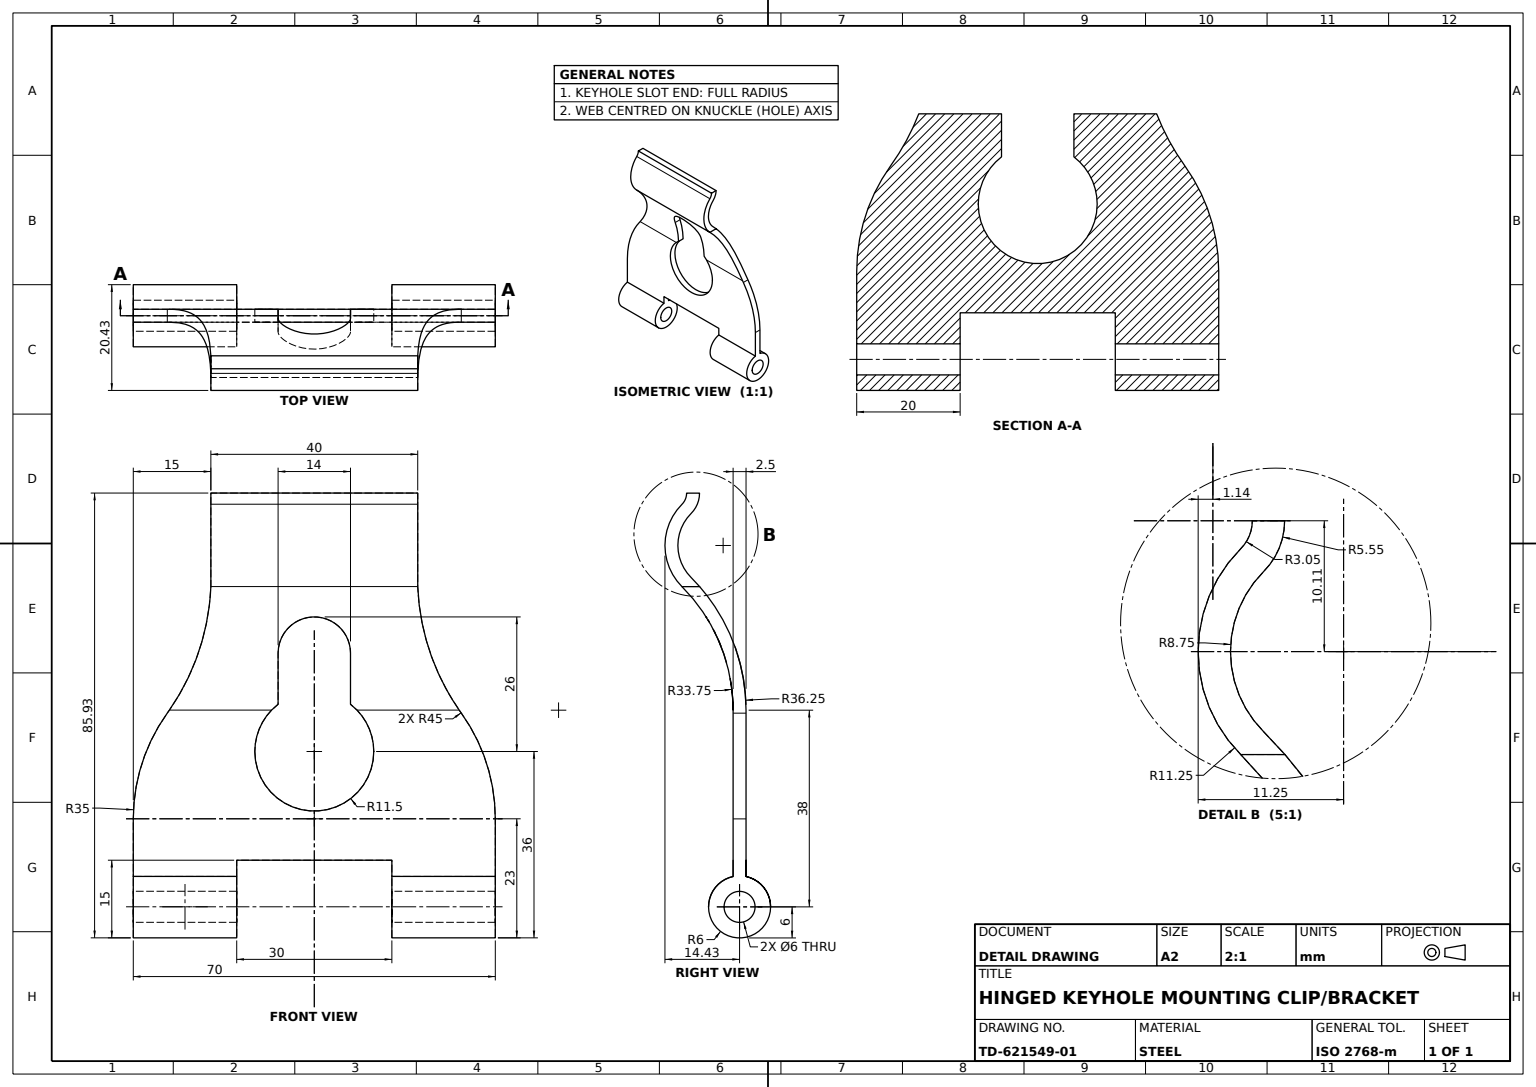
ISO-10303-21;
HEADER;
FILE_DESCRIPTION((''),'2;1');
FILE_NAME('','',(''),(''),'','','');
FILE_SCHEMA(('AUTOMOTIVE_DESIGN'));
ENDSEC;
DATA;
#1=APPLICATION_CONTEXT('');
#2=PRODUCT_CONTEXT('',#1,'mechanical');
#3=PRODUCT('','','',(#2));
#4=PRODUCT_DEFINITION_FORMATION('','',#3);
#5=PRODUCT_DEFINITION_CONTEXT('',#1,'design');
#6=PRODUCT_DEFINITION('','',#4,#5);
#7=PRODUCT_DEFINITION_SHAPE('','',#6);
#8=(LENGTH_UNIT()NAMED_UNIT(*)SI_UNIT(.MILLI.,.METRE.));
#9=(NAMED_UNIT(*)PLANE_ANGLE_UNIT()SI_UNIT($,.RADIAN.));
#10=(NAMED_UNIT(*)SI_UNIT($,.STERADIAN.)SOLID_ANGLE_UNIT());
#11=UNCERTAINTY_MEASURE_WITH_UNIT(LENGTH_MEASURE(1.E-05),#8,'distance_accuracy_value','');
#12=(GEOMETRIC_REPRESENTATION_CONTEXT(3)GLOBAL_UNCERTAINTY_ASSIGNED_CONTEXT((#11))GLOBAL_UNIT_ASSIGNED_CONTEXT((#8,#9,#10))REPRESENTATION_CONTEXT('',''));
#13=CARTESIAN_POINT('',(15.,0.,6.));
#14=VERTEX_POINT('',#13);
#15=CARTESIAN_POINT('',(15.,5.868347,1.25));
#16=VERTEX_POINT('',#15);
#17=CARTESIAN_POINT('',(15.,0.,0.));
#18=DIRECTION('',(-1.,0.,0.));
#19=DIRECTION('',(0.,-1.,0.));
#20=AXIS2_PLACEMENT_3D('',#17,#18,#19);
#21=CIRCLE('',#20,6.);
#22=EDGE_CURVE('',#14,#16,#21,.T.);
#23=ORIENTED_EDGE('',*,*,#22,.F.);
#24=CARTESIAN_POINT('',(35.,0.,6.));
#25=VERTEX_POINT('',#24);
#26=VECTOR('',#18,1000.);
#27=LINE('',#24,#26);
#28=EDGE_CURVE('',#25,#14,#27,.T.);
#29=ORIENTED_EDGE('',*,*,#28,.F.);
#30=CARTESIAN_POINT('',(35.,5.868347,1.25));
#31=VERTEX_POINT('',#30);
#32=CARTESIAN_POINT('',(35.,0.,0.));
#33=DIRECTION('',(1.,0.,0.));
#34=DIRECTION('',(0.,0.,-1.));
#35=AXIS2_PLACEMENT_3D('',#32,#33,#34);
#36=CIRCLE('',#35,6.);
#37=EDGE_CURVE('',#31,#25,#36,.T.);
#38=ORIENTED_EDGE('',*,*,#37,.F.);
#39=LINE('',#30,#26);
#40=EDGE_CURVE('',#31,#16,#39,.T.);
#41=ORIENTED_EDGE('',*,*,#40,.T.);
#42=EDGE_LOOP('',(#23,#29,#38,#41));
#43=FACE_OUTER_BOUND('',#42,.T.);
#44=DIRECTION('',(0.,0.,1.));
#45=AXIS2_PLACEMENT_3D('',#32,#18,#44);
#46=CYLINDRICAL_SURFACE('',#45,6.);
#47=ADVANCED_FACE('',(#43),#46,.T.);
#48=CARTESIAN_POINT('',(-15.,0.,-3.));
#49=VERTEX_POINT('',#48);
#50=CARTESIAN_POINT('',(-15.,0.,3.));
#51=VERTEX_POINT('',#50);
#52=CARTESIAN_POINT('',(-15.,0.,0.));
#53=AXIS2_PLACEMENT_3D('',#52,#33,#34);
#54=CIRCLE('',#53,3.);
#55=EDGE_CURVE('',#49,#51,#54,.T.);
#56=ORIENTED_EDGE('',*,*,#55,.F.);
#57=EDGE_CURVE('',#51,#49,#54,.T.);
#58=ORIENTED_EDGE('',*,*,#57,.F.);
#59=EDGE_LOOP('',(#56,#58));
#60=FACE_BOUND('',#59,.T.);
#61=CARTESIAN_POINT('',(-15.,5.868347,1.25));
#62=VERTEX_POINT('',#61);
#63=CARTESIAN_POINT('',(-15.,0.,6.));
#64=VERTEX_POINT('',#63);
#65=CIRCLE('',#53,6.);
#66=EDGE_CURVE('',#62,#64,#65,.T.);
#67=ORIENTED_EDGE('',*,*,#66,.T.);
#68=CARTESIAN_POINT('',(-15.,0.,-6.));
#69=VERTEX_POINT('',#68);
#70=EDGE_CURVE('',#64,#69,#65,.T.);
#71=ORIENTED_EDGE('',*,*,#70,.T.);
#72=CARTESIAN_POINT('',(-15.,5.868347,-1.25));
#73=VERTEX_POINT('',#72);
#74=EDGE_CURVE('',#69,#73,#65,.T.);
#75=ORIENTED_EDGE('',*,*,#74,.T.);
#76=CARTESIAN_POINT('',(-15.,9.,-1.25));
#77=VERTEX_POINT('',#76);
#78=DIRECTION('',(0.,1.,0.));
#79=VECTOR('',#78,1000.);
#80=LINE('',#72,#79);
#81=EDGE_CURVE('',#73,#77,#80,.T.);
#82=ORIENTED_EDGE('',*,*,#81,.T.);
#83=CARTESIAN_POINT('',(-15.,9.,1.25));
#84=VERTEX_POINT('',#83);
#85=CARTESIAN_POINT('',(-15.,9.,-6.));
#86=VECTOR('',#44,1000.);
#87=LINE('',#85,#86);
#88=EDGE_CURVE('',#77,#84,#87,.T.);
#89=ORIENTED_EDGE('',*,*,#88,.T.);
#90=VECTOR('',#19,1000.);
#91=LINE('',#61,#90);
#92=EDGE_CURVE('',#84,#62,#91,.T.);
#93=ORIENTED_EDGE('',*,*,#92,.T.);
#94=EDGE_LOOP('',(#67,#71,#75,#82,#89,#93));
#95=FACE_OUTER_BOUND('',#94,.T.);
#96=CARTESIAN_POINT('',(-15.,-6.,-6.));
#97=AXIS2_PLACEMENT_3D('',#96,#33,#34);
#98=PLANE('',#97);
#99=ADVANCED_FACE('',(#60,#95),#98,.T.);
#100=ORIENTED_EDGE('',*,*,#70,.F.);
#101=CARTESIAN_POINT('',(-35.,0.,6.));
#102=VERTEX_POINT('',#101);
#103=EDGE_CURVE('',#64,#102,#27,.T.);
#104=ORIENTED_EDGE('',*,*,#103,.T.);
#105=CARTESIAN_POINT('',(-35.,0.,-6.));
#106=VERTEX_POINT('',#105);
#107=CARTESIAN_POINT('',(-35.,0.,0.));
#108=AXIS2_PLACEMENT_3D('',#107,#33,#34);
#109=CIRCLE('',#108,6.);
#110=EDGE_CURVE('',#102,#106,#109,.T.);
#111=ORIENTED_EDGE('',*,*,#110,.T.);
#112=CARTESIAN_POINT('',(35.,0.,-6.));
#113=LINE('',#112,#26);
#114=EDGE_CURVE('',#69,#106,#113,.T.);
#115=ORIENTED_EDGE('',*,*,#114,.F.);
#116=EDGE_LOOP('',(#100,#104,#111,#115));
#117=FACE_OUTER_BOUND('',#116,.T.);
#118=ADVANCED_FACE('',(#117),#46,.T.);
#119=CARTESIAN_POINT('',(7.,49.,3.092908));
#120=VERTEX_POINT('',#119);
#121=CARTESIAN_POINT('',(7.,39.124144,1.268727));
#122=VERTEX_POINT('',#121);
#123=CARTESIAN_POINT('',(7.,38.,35.));
#124=AXIS2_PLACEMENT_3D('',#123,#18,#78);
#125=CIRCLE('',#124,33.75);
#126=EDGE_CURVE('',#120,#122,#125,.T.);
#127=ORIENTED_EDGE('',*,*,#126,.T.);
#128=CARTESIAN_POINT('',(8.261356,38.,1.25));
#129=VERTEX_POINT('',#128);
#130=CARTESIAN_POINT('',(7.448007,38.780435,1.257272));
#131=CARTESIAN_POINT('',(7.868457,38.405735,1.25));
#132=B_SPLINE_CURVE_WITH_KNOTS('',3,(#121,#130,#131,#128),.UNSPECIFIED.,.F.,.F.,(4,4),(0.,0.001689695),.UNSPECIFIED.);
#133=EDGE_CURVE('',#122,#129,#132,.T.);
#134=ORIENTED_EDGE('',*,*,#133,.T.);
#135=CARTESIAN_POINT('',(28.015673,38.,1.25));
#136=VERTEX_POINT('',#135);
#137=CARTESIAN_POINT('',(35.,38.,1.25));
#138=LINE('',#137,#26);
#139=EDGE_CURVE('',#136,#129,#138,.T.);
#140=ORIENTED_EDGE('',*,*,#139,.F.);
#141=CARTESIAN_POINT('',(20.,61.864854,11.135146));
#142=VERTEX_POINT('',#141);
#143=CARTESIAN_POINT('',(20.067704,60.195455,9.465747));
#144=CARTESIAN_POINT('',(20.233479,58.385184,8.002505));
#145=CARTESIAN_POINT('',(20.628542,55.962208,6.421049));
#146=CARTESIAN_POINT('',(20.717007,55.469533,6.117247));
#147=CARTESIAN_POINT('',(20.914793,54.468142,5.534795));
#148=CARTESIAN_POINT('',(21.024568,53.957601,5.255257));
#149=CARTESIAN_POINT('',(21.38398,52.420105,4.463923));
#150=CARTESIAN_POINT('',(21.663718,51.385624,3.997756));
#151=CARTESIAN_POINT('',(22.310298,49.303225,3.179391));
#152=CARTESIAN_POINT('',(22.677119,48.255291,2.827222));
#153=CARTESIAN_POINT('',(23.298532,46.676942,2.37988));
#154=CARTESIAN_POINT('',(23.517542,46.149748,2.24427));
#155=CARTESIAN_POINT('',(23.980432,45.09379,1.999479));
#156=CARTESIAN_POINT('',(24.224013,44.565913,1.890595));
#157=CARTESIAN_POINT('',(25.490165,41.956451,1.415609));
#158=CARTESIAN_POINT('',(26.66763,39.93888,1.25));
#159=B_SPLINE_CURVE_WITH_KNOTS('',3,(#141,#143,#144,#145,#146,#147,#148,#149,#150,#151,#152,#153,#154,#155,#156,#157,#158,#135),.UNSPECIFIED.,.F.,.F.,(4,2,2,2,2,2,2,2,4),(0.,0.006991698,0.008739623,0.010487547,0.013983397,0.017479246,0.01922717,0.020975095,0.027966793),.UNSPECIFIED.);
#160=EDGE_CURVE('',#142,#136,#159,.T.);
#161=ORIENTED_EDGE('',*,*,#160,.F.);
#162=CARTESIAN_POINT('',(-20.,61.864854,11.135146));
#163=VERTEX_POINT('',#162);
#164=CARTESIAN_POINT('',(35.,61.864854,11.135146));
#165=LINE('',#164,#26);
#166=EDGE_CURVE('',#142,#163,#165,.T.);
#167=ORIENTED_EDGE('',*,*,#166,.T.);
#168=CARTESIAN_POINT('',(-28.015673,38.,1.25));
#169=VERTEX_POINT('',#168);
#170=CARTESIAN_POINT('',(-26.66803,39.938305,1.25));
#171=CARTESIAN_POINT('',(-25.494861,41.949522,1.415707));
#172=CARTESIAN_POINT('',(-24.235569,44.541424,1.885806));
#173=CARTESIAN_POINT('',(-23.994118,45.063713,1.993062));
#174=CARTESIAN_POINT('',(-23.531942,46.115821,2.235882));
#175=CARTESIAN_POINT('',(-23.310498,46.647516,2.371999));
#176=CARTESIAN_POINT('',(-22.683251,48.237849,2.821393));
#177=CARTESIAN_POINT('',(-22.314887,49.289626,3.174576));
#178=CARTESIAN_POINT('',(-21.667657,51.371771,3.991791));
#179=CARTESIAN_POINT('',(-21.388816,52.402154,4.455803));
#180=CARTESIAN_POINT('',(-21.031209,53.927873,5.239418));
#181=CARTESIAN_POINT('',(-20.922125,54.43313,5.515242));
#182=CARTESIAN_POINT('',(-20.723185,55.436284,6.09715));
#183=CARTESIAN_POINT('',(-20.633244,55.935017,6.403886));
#184=CARTESIAN_POINT('',(-20.233612,58.377977,7.99553));
#185=CARTESIAN_POINT('',(-20.067728,60.194856,9.465148));
#186=B_SPLINE_CURVE_WITH_KNOTS('',3,(#168,#170,#171,#172,#173,#174,#175,#176,#177,#178,#179,#180,#181,#182,#183,#184,#185,#162),.UNSPECIFIED.,.F.,.F.,(4,2,2,2,2,2,2,2,4),(0.,0.006992736,0.00874092,0.010489104,0.013985472,0.01748184,0.019230024,0.020978208,0.027970943),.UNSPECIFIED.);
#187=EDGE_CURVE('',#169,#163,#186,.T.);
#188=ORIENTED_EDGE('',*,*,#187,.F.);
#189=CARTESIAN_POINT('',(-8.261356,38.,1.25));
#190=VERTEX_POINT('',#189);
#191=EDGE_CURVE('',#190,#169,#138,.T.);
#192=ORIENTED_EDGE('',*,*,#191,.F.);
#193=CARTESIAN_POINT('',(-7.,39.124144,1.268727));
#194=VERTEX_POINT('',#193);
#195=CARTESIAN_POINT('',(-7.868457,38.405735,1.25));
#196=CARTESIAN_POINT('',(-7.448007,38.780435,1.257272));
#197=B_SPLINE_CURVE_WITH_KNOTS('',3,(#189,#195,#196,#193),.UNSPECIFIED.,.F.,.F.,(4,4),(0.,0.001689695),.UNSPECIFIED.);
#198=EDGE_CURVE('',#190,#194,#197,.T.);
#199=ORIENTED_EDGE('',*,*,#198,.T.);
#200=CARTESIAN_POINT('',(-7.,49.,3.092908));
#201=VERTEX_POINT('',#200);
#202=CARTESIAN_POINT('',(-7.,38.,35.));
#203=AXIS2_PLACEMENT_3D('',#202,#33,#19);
#204=CIRCLE('',#203,33.75);
#205=EDGE_CURVE('',#194,#201,#204,.T.);
#206=ORIENTED_EDGE('',*,*,#205,.T.);
#207=CARTESIAN_POINT('',(-7.,49.459493,3.251319));
#208=CARTESIAN_POINT('',(-6.955225,49.908016,3.417036));
#209=CARTESIAN_POINT('',(-6.826304,50.565722,3.675559));
#210=CARTESIAN_POINT('',(-6.772953,50.78243,3.763389));
#211=CARTESIAN_POINT('',(-6.645453,51.210861,3.942158));
#212=CARTESIAN_POINT('',(-6.570874,51.423584,4.033545));
#213=CARTESIAN_POINT('',(-6.31836,52.046131,4.308397));
#214=CARTESIAN_POINT('',(-6.11307,52.439076,4.491852));
#215=CARTESIAN_POINT('',(-5.750706,52.997324,4.764496));
#216=CARTESIAN_POINT('',(-5.620776,53.178174,4.854944));
#217=CARTESIAN_POINT('',(-5.341893,53.529287,5.03431));
#218=CARTESIAN_POINT('',(-5.192379,53.699984,5.123477));
#219=CARTESIAN_POINT('',(-4.723451,54.185711,5.382103));
#220=CARTESIAN_POINT('',(-4.381504,54.478099,5.544528));
#221=CARTESIAN_POINT('',(-3.821821,54.869026,5.767809));
#222=CARTESIAN_POINT('',(-3.627407,54.991332,5.838817));
#223=CARTESIAN_POINT('',(-3.221534,55.218992,5.972664));
#224=CARTESIAN_POINT('',(-3.010536,55.323866,6.035227));
#225=CARTESIAN_POINT('',(-2.367891,55.6039,6.203946));
#226=CARTESIAN_POINT('',(-1.921495,55.747942,6.29309));
#227=CARTESIAN_POINT('',(-1.222655,55.896509,6.385653));
#228=CARTESIAN_POINT('',(-0.983157,55.934845,6.409708));
#229=CARTESIAN_POINT('',(-0.501467,55.986215,6.441998));
#230=CARTESIAN_POINT('',(-0.26109,55.999242,6.450223));
#231=CARTESIAN_POINT('',(0.21875,56.000694,6.451138));
#232=CARTESIAN_POINT('',(0.458214,55.989116,6.443827));
#233=CARTESIAN_POINT('',(0.936227,55.941266,6.41374));
#234=CARTESIAN_POINT('',(1.176202,55.904679,6.390766));
#235=CARTESIAN_POINT('',(1.884086,55.758874,6.29986));
#236=CARTESIAN_POINT('',(2.335046,55.615791,6.211226));
#237=CARTESIAN_POINT('',(2.982968,55.33697,6.043071));
#238=CARTESIAN_POINT('',(3.195077,55.232627,5.980761));
#239=CARTESIAN_POINT('',(3.601997,55.006645,5.847749));
#240=CARTESIAN_POINT('',(3.797576,54.884796,5.776915));
#241=CARTESIAN_POINT('',(4.173959,54.624098,5.627829));
#242=CARTESIAN_POINT('',(4.35476,54.485245,5.549575));
#243=CARTESIAN_POINT('',(4.702032,54.19064,5.386591));
#244=CARTESIAN_POINT('',(4.869045,54.034225,5.301517));
#245=CARTESIAN_POINT('',(5.340682,53.547659,5.042231));
#246=CARTESIAN_POINT('',(5.618752,53.19864,4.863034));
#247=CARTESIAN_POINT('',(6.106229,52.451511,4.497717));
#248=CARTESIAN_POINT('',(6.315978,52.050643,4.310508));
#249=CARTESIAN_POINT('',(6.651425,51.226332,3.946342));
#250=CARTESIAN_POINT('',(6.779579,50.799961,3.767828));
#251=CARTESIAN_POINT('',(6.954259,49.916967,3.420362));
#252=CARTESIAN_POINT('',(7.,49.46001,3.251497));
#253=B_SPLINE_CURVE_WITH_KNOTS('',3,(#200,#207,#208,#209,#210,#211,#212,#213,#214,#215,#216,#217,#218,#219,#220,#221,#222,#223,#224,#225,#226,#227,#228,#229,#230,#231,#232,#233,#234,#235,#236,#237,#238,#239,#240,#241,#242,#243,#244,#245,#246,#247,#248,#249,#250,#251,#252,#119),.UNSPECIFIED.,.F.,.F.,(4,2,2,2,2,2,2,2,2,2,2,2,2,2,2,2,2,2,2,2,2,2,2,4),(0.,0.00143658,0.00215487,0.00287316,0.004309739,0.005028029,0.005746319,0.007182899,0.007901189,0.008619479,0.010056058,0.010774348,0.011492638,0.012210928,0.012929218,0.014365798,0.015084088,0.015802378,0.016520667,0.017238957,0.018675537,0.020112117,0.021548697,0.022985276),.UNSPECIFIED.);
#254=EDGE_CURVE('',#201,#120,#253,.T.);
#255=ORIENTED_EDGE('',*,*,#254,.T.);
#256=EDGE_LOOP('',(#127,#134,#140,#161,#167,#188,#192,#199,#206,#255));
#257=FACE_OUTER_BOUND('',#256,.T.);
#258=CARTESIAN_POINT('',(35.,38.,35.));
#259=AXIS2_PLACEMENT_3D('',#258,#18,#44);
#260=CYLINDRICAL_SURFACE('',#259,33.75);
#261=ADVANCED_FACE('',(#257),#260,.F.);
#262=CARTESIAN_POINT('',(-20.,77.774756,11.135146));
#263=VERTEX_POINT('',#262);
#264=CARTESIAN_POINT('',(-20.,79.931432,10.241822));
#265=VERTEX_POINT('',#264);
#266=CARTESIAN_POINT('',(-20.,79.931432,13.291822));
#267=AXIS2_PLACEMENT_3D('',#266,#33,#19);
#268=CIRCLE('',#267,3.05);
#269=EDGE_CURVE('',#263,#265,#268,.T.);
#270=ORIENTED_EDGE('',*,*,#269,.F.);
#271=CARTESIAN_POINT('',(20.,77.774756,11.135146));
#272=VERTEX_POINT('',#271);
#273=CARTESIAN_POINT('',(35.,77.774756,11.135146));
#274=LINE('',#273,#26);
#275=EDGE_CURVE('',#272,#263,#274,.T.);
#276=ORIENTED_EDGE('',*,*,#275,.F.);
#277=CARTESIAN_POINT('',(20.,79.931432,10.241822));
#278=VERTEX_POINT('',#277);
#279=CARTESIAN_POINT('',(20.,79.931432,13.291822));
#280=AXIS2_PLACEMENT_3D('',#279,#18,#34);
#281=CIRCLE('',#280,3.05);
#282=EDGE_CURVE('',#278,#272,#281,.T.);
#283=ORIENTED_EDGE('',*,*,#282,.F.);
#284=CARTESIAN_POINT('',(35.,79.931432,10.241822));
#285=LINE('',#284,#26);
#286=EDGE_CURVE('',#278,#265,#285,.T.);
#287=ORIENTED_EDGE('',*,*,#286,.T.);
#288=EDGE_LOOP('',(#270,#276,#283,#287));
#289=FACE_OUTER_BOUND('',#288,.T.);
#290=CARTESIAN_POINT('',(35.,79.931432,13.291822));
#291=AXIS2_PLACEMENT_3D('',#290,#18,#44);
#292=CYLINDRICAL_SURFACE('',#291,3.05);
#293=ADVANCED_FACE('',(#289),#292,.F.);
#294=CARTESIAN_POINT('',(28.421329,37.426161,1.25));
#295=VERTEX_POINT('',#294);
#296=CARTESIAN_POINT('',(35.,17.,1.25));
#297=VERTEX_POINT('',#296);
#298=CARTESIAN_POINT('',(0.,17.,1.25));
#299=AXIS2_PLACEMENT_3D('',#298,#34,#78);
#300=CIRCLE('',#299,35.);
#301=EDGE_CURVE('',#295,#297,#300,.T.);
#302=ORIENTED_EDGE('',*,*,#301,.T.);
#303=CARTESIAN_POINT('',(35.,17.,-1.25));
#304=VERTEX_POINT('',#303);
#305=CARTESIAN_POINT('',(35.,17.,-6.));
#306=LINE('',#305,#86);
#307=EDGE_CURVE('',#304,#297,#306,.T.);
#308=ORIENTED_EDGE('',*,*,#307,.F.);
#309=CARTESIAN_POINT('',(28.421329,37.426161,-1.25));
#310=VERTEX_POINT('',#309);
#311=CARTESIAN_POINT('',(0.,17.,-1.25));
#312=AXIS2_PLACEMENT_3D('',#311,#44,#19);
#313=CIRCLE('',#312,35.);
#314=EDGE_CURVE('',#304,#310,#313,.T.);
#315=ORIENTED_EDGE('',*,*,#314,.T.);
#316=CARTESIAN_POINT('',(28.421329,37.426161,-6.));
#317=LINE('',#316,#86);
#318=EDGE_CURVE('',#310,#295,#317,.T.);
#319=ORIENTED_EDGE('',*,*,#318,.T.);
#320=EDGE_LOOP('',(#302,#308,#315,#319));
#321=FACE_OUTER_BOUND('',#320,.T.);
#322=CARTESIAN_POINT('',(0.,17.,-6.));
#323=AXIS2_PLACEMENT_3D('',#322,#44,#33);
#324=CYLINDRICAL_SURFACE('',#323,35.);
#325=ADVANCED_FACE('',(#321),#324,.T.);
#326=CARTESIAN_POINT('',(-35.,0.,-3.));
#327=VERTEX_POINT('',#326);
#328=CARTESIAN_POINT('',(-35.,0.,3.));
#329=VERTEX_POINT('',#328);
#330=CIRCLE('',#108,3.);
#331=EDGE_CURVE('',#327,#329,#330,.T.);
#332=ORIENTED_EDGE('',*,*,#331,.F.);
#333=CARTESIAN_POINT('',(35.,0.,-3.));
#334=LINE('',#333,#26);
#335=EDGE_CURVE('',#49,#327,#334,.T.);
#336=ORIENTED_EDGE('',*,*,#335,.F.);
#337=ORIENTED_EDGE('',*,*,#55,.T.);
#338=CARTESIAN_POINT('',(35.,0.,3.));
#339=LINE('',#338,#26);
#340=EDGE_CURVE('',#51,#329,#339,.T.);
#341=ORIENTED_EDGE('',*,*,#340,.T.);
#342=EDGE_LOOP('',(#332,#336,#337,#341));
#343=FACE_OUTER_BOUND('',#342,.T.);
#344=CYLINDRICAL_SURFACE('',#45,3.);
#345=ADVANCED_FACE('',(#343),#344,.F.);
#346=CARTESIAN_POINT('',(20.,76.006989,9.367379));
#347=VERTEX_POINT('',#346);
#348=CARTESIAN_POINT('',(-20.,76.006989,9.367379));
#349=VERTEX_POINT('',#348);
#350=CARTESIAN_POINT('',(35.,76.006989,9.367379));
#351=LINE('',#350,#26);
#352=EDGE_CURVE('',#347,#349,#351,.T.);
#353=ORIENTED_EDGE('',*,*,#352,.T.);
#354=CARTESIAN_POINT('',(-20.,79.931432,7.741822));
#355=VERTEX_POINT('',#354);
#356=AXIS2_PLACEMENT_3D('',#266,#18,#19);
#357=CIRCLE('',#356,5.55);
#358=EDGE_CURVE('',#355,#349,#357,.T.);
#359=ORIENTED_EDGE('',*,*,#358,.F.);
#360=CARTESIAN_POINT('',(20.,79.931432,7.741822));
#361=VERTEX_POINT('',#360);
#362=CARTESIAN_POINT('',(35.,79.931432,7.741822));
#363=LINE('',#362,#26);
#364=EDGE_CURVE('',#361,#355,#363,.T.);
#365=ORIENTED_EDGE('',*,*,#364,.F.);
#366=AXIS2_PLACEMENT_3D('',#279,#33,#34);
#367=CIRCLE('',#366,5.55);
#368=EDGE_CURVE('',#347,#361,#367,.T.);
#369=ORIENTED_EDGE('',*,*,#368,.F.);
#370=EDGE_LOOP('',(#353,#359,#365,#369));
#371=FACE_OUTER_BOUND('',#370,.T.);
#372=CYLINDRICAL_SURFACE('',#291,5.55);
#373=ADVANCED_FACE('',(#371),#372,.T.);
#374=CARTESIAN_POINT('',(-20.,69.819805,11.930195));
#375=VERTEX_POINT('',#374);
#376=CARTESIAN_POINT('',(-20.,69.819805,3.180195));
#377=AXIS2_PLACEMENT_3D('',#376,#33,#19);
#378=CIRCLE('',#377,8.75);
#379=EDGE_CURVE('',#349,#375,#378,.T.);
#380=ORIENTED_EDGE('',*,*,#379,.F.);
#381=ORIENTED_EDGE('',*,*,#352,.F.);
#382=CARTESIAN_POINT('',(20.,69.819805,11.930195));
#383=VERTEX_POINT('',#382);
#384=CARTESIAN_POINT('',(20.,69.819805,3.180195));
#385=AXIS2_PLACEMENT_3D('',#384,#18,#34);
#386=CIRCLE('',#385,8.75);
#387=EDGE_CURVE('',#383,#347,#386,.T.);
#388=ORIENTED_EDGE('',*,*,#387,.F.);
#389=CARTESIAN_POINT('',(35.,69.819805,11.930195));
#390=LINE('',#389,#26);
#391=EDGE_CURVE('',#383,#375,#390,.T.);
#392=ORIENTED_EDGE('',*,*,#391,.T.);
#393=EDGE_LOOP('',(#380,#381,#388,#392));
#394=FACE_OUTER_BOUND('',#393,.T.);
#395=CARTESIAN_POINT('',(35.,69.819805,3.180195));
#396=AXIS2_PLACEMENT_3D('',#395,#18,#44);
#397=CYLINDRICAL_SURFACE('',#396,8.75);
#398=ADVANCED_FACE('',(#394),#397,.F.);
#399=CARTESIAN_POINT('',(20.,69.819805,14.430195));
#400=VERTEX_POINT('',#399);
#401=AXIS2_PLACEMENT_3D('',#384,#33,#34);
#402=CIRCLE('',#401,11.25);
#403=EDGE_CURVE('',#400,#142,#402,.T.);
#404=ORIENTED_EDGE('',*,*,#403,.F.);
#405=CARTESIAN_POINT('',(-20.,69.819805,14.430195));
#406=VERTEX_POINT('',#405);
#407=CARTESIAN_POINT('',(35.,69.819805,14.430195));
#408=LINE('',#407,#26);
#409=EDGE_CURVE('',#400,#406,#408,.T.);
#410=ORIENTED_EDGE('',*,*,#409,.T.);
#411=AXIS2_PLACEMENT_3D('',#376,#18,#19);
#412=CIRCLE('',#411,11.25);
#413=EDGE_CURVE('',#163,#406,#412,.T.);
#414=ORIENTED_EDGE('',*,*,#413,.F.);
#415=ORIENTED_EDGE('',*,*,#166,.F.);
#416=EDGE_LOOP('',(#404,#410,#414,#415));
#417=FACE_OUTER_BOUND('',#416,.T.);
#418=CYLINDRICAL_SURFACE('',#396,11.25);
#419=ADVANCED_FACE('',(#417),#418,.T.);
#420=ORIENTED_EDGE('',*,*,#88,.F.);
#421=CARTESIAN_POINT('',(15.,9.,-1.25));
#422=VERTEX_POINT('',#421);
#423=CARTESIAN_POINT('',(35.,9.,-1.25));
#424=VECTOR('',#33,1000.);
#425=LINE('',#423,#424);
#426=EDGE_CURVE('',#77,#422,#425,.T.);
#427=ORIENTED_EDGE('',*,*,#426,.T.);
#428=CARTESIAN_POINT('',(15.,9.,1.25));
#429=VERTEX_POINT('',#428);
#430=CARTESIAN_POINT('',(15.,9.,-6.));
#431=LINE('',#430,#86);
#432=EDGE_CURVE('',#422,#429,#431,.T.);
#433=ORIENTED_EDGE('',*,*,#432,.T.);
#434=CARTESIAN_POINT('',(35.,9.,1.25));
#435=LINE('',#434,#26);
#436=EDGE_CURVE('',#429,#84,#435,.T.);
#437=ORIENTED_EDGE('',*,*,#436,.T.);
#438=EDGE_LOOP('',(#420,#427,#433,#437));
#439=FACE_OUTER_BOUND('',#438,.T.);
#440=AXIS2_PLACEMENT_3D('',#85,#19,#33);
#441=PLANE('',#440);
#442=ADVANCED_FACE('',(#439),#441,.T.);
#443=VERTEX_POINT('',#338);
#444=VERTEX_POINT('',#333);
#445=CIRCLE('',#35,3.);
#446=EDGE_CURVE('',#443,#444,#445,.T.);
#447=ORIENTED_EDGE('',*,*,#446,.T.);
#448=CARTESIAN_POINT('',(15.,0.,-3.));
#449=VERTEX_POINT('',#448);
#450=EDGE_CURVE('',#444,#449,#334,.T.);
#451=ORIENTED_EDGE('',*,*,#450,.T.);
#452=CARTESIAN_POINT('',(15.,0.,3.));
#453=VERTEX_POINT('',#452);
#454=CIRCLE('',#20,3.);
#455=EDGE_CURVE('',#449,#453,#454,.T.);
#456=ORIENTED_EDGE('',*,*,#455,.T.);
#457=EDGE_CURVE('',#443,#453,#339,.T.);
#458=ORIENTED_EDGE('',*,*,#457,.F.);
#459=EDGE_LOOP('',(#447,#451,#456,#458));
#460=FACE_OUTER_BOUND('',#459,.T.);
#461=ADVANCED_FACE('',(#460),#344,.F.);
#462=CARTESIAN_POINT('',(-35.,5.868347,1.25));
#463=VERTEX_POINT('',#462);
#464=EDGE_CURVE('',#62,#463,#39,.T.);
#465=ORIENTED_EDGE('',*,*,#464,.F.);
#466=ORIENTED_EDGE('',*,*,#92,.F.);
#467=ORIENTED_EDGE('',*,*,#436,.F.);
#468=LINE('',#15,#79);
#469=EDGE_CURVE('',#16,#429,#468,.T.);
#470=ORIENTED_EDGE('',*,*,#469,.F.);
#471=ORIENTED_EDGE('',*,*,#40,.F.);
#472=LINE('',#30,#90);
#473=EDGE_CURVE('',#297,#31,#472,.T.);
#474=ORIENTED_EDGE('',*,*,#473,.F.);
#475=ORIENTED_EDGE('',*,*,#301,.F.);
#476=CARTESIAN_POINT('',(64.963038,63.688368,1.25));
#477=AXIS2_PLACEMENT_3D('',#476,#44,#78);
#478=CIRCLE('',#477,45.);
#479=EDGE_CURVE('',#136,#295,#478,.T.);
#480=ORIENTED_EDGE('',*,*,#479,.F.);
#481=ORIENTED_EDGE('',*,*,#139,.T.);
#482=CARTESIAN_POINT('',(11.5,30.,1.25));
#483=VERTEX_POINT('',#482);
#484=CARTESIAN_POINT('',(0.,30.,1.25));
#485=AXIS2_PLACEMENT_3D('',#484,#34,#78);
#486=CIRCLE('',#485,11.5);
#487=EDGE_CURVE('',#129,#483,#486,.T.);
#488=ORIENTED_EDGE('',*,*,#487,.T.);
#489=CARTESIAN_POINT('',(-11.5,30.,1.25));
#490=VERTEX_POINT('',#489);
#491=EDGE_CURVE('',#483,#490,#486,.T.);
#492=ORIENTED_EDGE('',*,*,#491,.T.);
#493=EDGE_CURVE('',#490,#190,#486,.T.);
#494=ORIENTED_EDGE('',*,*,#493,.T.);
#495=ORIENTED_EDGE('',*,*,#191,.T.);
#496=CARTESIAN_POINT('',(-28.421329,37.426161,1.25));
#497=VERTEX_POINT('',#496);
#498=CARTESIAN_POINT('',(-64.963038,63.688368,1.25));
#499=AXIS2_PLACEMENT_3D('',#498,#44,#78);
#500=CIRCLE('',#499,45.);
#501=EDGE_CURVE('',#497,#169,#500,.T.);
#502=ORIENTED_EDGE('',*,*,#501,.F.);
#503=CARTESIAN_POINT('',(-35.,17.,1.25));
#504=VERTEX_POINT('',#503);
#505=EDGE_CURVE('',#504,#497,#300,.T.);
#506=ORIENTED_EDGE('',*,*,#505,.F.);
#507=LINE('',#462,#90);
#508=EDGE_CURVE('',#504,#463,#507,.T.);
#509=ORIENTED_EDGE('',*,*,#508,.T.);
#510=EDGE_LOOP('',(#465,#466,#467,#470,#471,#474,#475,#480,#481,#488,#492,#494,#495,#502,#506,#509));
#511=FACE_OUTER_BOUND('',#510,.T.);
#512=AXIS2_PLACEMENT_3D('',#30,#34,#78);
#513=PLANE('',#512);
#514=ADVANCED_FACE('',(#511),#513,.F.);
#515=CARTESIAN_POINT('',(-7.,39.124144,-1.232565));
#516=VERTEX_POINT('',#515);
#517=CARTESIAN_POINT('',(-7.,39.124144,-6.));
#518=LINE('',#517,#86);
#519=EDGE_CURVE('',#516,#194,#518,.T.);
#520=ORIENTED_EDGE('',*,*,#519,.F.);
#521=CARTESIAN_POINT('',(-7.,49.,0.459263));
#522=VERTEX_POINT('',#521);
#523=AXIS2_PLACEMENT_3D('',#202,#18,#19);
#524=CIRCLE('',#523,36.25);
#525=EDGE_CURVE('',#522,#516,#524,.T.);
#526=ORIENTED_EDGE('',*,*,#525,.F.);
#527=CARTESIAN_POINT('',(-7.,49.,-6.));
#528=LINE('',#527,#86);
#529=EDGE_CURVE('',#522,#201,#528,.T.);
#530=ORIENTED_EDGE('',*,*,#529,.T.);
#531=ORIENTED_EDGE('',*,*,#205,.F.);
#532=EDGE_LOOP('',(#520,#526,#530,#531));
#533=FACE_OUTER_BOUND('',#532,.T.);
#534=AXIS2_PLACEMENT_3D('',#527,#18,#19);
#535=PLANE('',#534);
#536=ADVANCED_FACE('',(#533),#535,.F.);
#537=ORIENTED_EDGE('',*,*,#282,.T.);
#538=EDGE_CURVE('',#272,#400,#402,.T.);
#539=ORIENTED_EDGE('',*,*,#538,.T.);
#540=ORIENTED_EDGE('',*,*,#403,.T.);
#541=CARTESIAN_POINT('',(20.,61.864854,7.7139));
#542=VERTEX_POINT('',#541);
#543=CARTESIAN_POINT('',(20.,61.864854,-6.));
#544=LINE('',#543,#86);
#545=EDGE_CURVE('',#542,#142,#544,.T.);
#546=ORIENTED_EDGE('',*,*,#545,.F.);
#547=CARTESIAN_POINT('',(20.,63.632621,9.367379));
#548=VERTEX_POINT('',#547);
#549=CARTESIAN_POINT('',(20.,38.,35.));
#550=AXIS2_PLACEMENT_3D('',#549,#33,#34);
#551=CIRCLE('',#550,36.25);
#552=EDGE_CURVE('',#542,#548,#551,.T.);
#553=ORIENTED_EDGE('',*,*,#552,.T.);
#554=EDGE_CURVE('',#548,#383,#386,.T.);
#555=ORIENTED_EDGE('',*,*,#554,.T.);
#556=ORIENTED_EDGE('',*,*,#387,.T.);
#557=ORIENTED_EDGE('',*,*,#368,.T.);
#558=CARTESIAN_POINT('',(20.,79.931432,-6.));
#559=LINE('',#558,#86);
#560=EDGE_CURVE('',#361,#278,#559,.T.);
#561=ORIENTED_EDGE('',*,*,#560,.T.);
#562=EDGE_LOOP('',(#537,#539,#540,#546,#553,#555,#556,#557,#561));
#563=FACE_OUTER_BOUND('',#562,.T.);
#564=AXIS2_PLACEMENT_3D('',#543,#33,#34);
#565=PLANE('',#564);
#566=ADVANCED_FACE('',(#563),#565,.T.);
#567=CARTESIAN_POINT('',(35.,5.868347,-1.25));
#568=VERTEX_POINT('',#567);
#569=CARTESIAN_POINT('',(15.,5.868347,-1.25));
#570=VERTEX_POINT('',#569);
#571=LINE('',#567,#26);
#572=EDGE_CURVE('',#568,#570,#571,.T.);
#573=ORIENTED_EDGE('',*,*,#572,.F.);
#574=VERTEX_POINT('',#112);
#575=EDGE_CURVE('',#574,#568,#36,.T.);
#576=ORIENTED_EDGE('',*,*,#575,.F.);
#577=CARTESIAN_POINT('',(15.,0.,-6.));
#578=VERTEX_POINT('',#577);
#579=EDGE_CURVE('',#574,#578,#113,.T.);
#580=ORIENTED_EDGE('',*,*,#579,.T.);
#581=EDGE_CURVE('',#570,#578,#21,.T.);
#582=ORIENTED_EDGE('',*,*,#581,.F.);
#583=EDGE_LOOP('',(#573,#576,#580,#582));
#584=FACE_OUTER_BOUND('',#583,.T.);
#585=ADVANCED_FACE('',(#584),#46,.T.);
#586=ORIENTED_EDGE('',*,*,#464,.T.);
#587=EDGE_CURVE('',#463,#102,#109,.T.);
#588=ORIENTED_EDGE('',*,*,#587,.T.);
#589=ORIENTED_EDGE('',*,*,#103,.F.);
#590=ORIENTED_EDGE('',*,*,#66,.F.);
#591=EDGE_LOOP('',(#586,#588,#589,#590));
#592=FACE_OUTER_BOUND('',#591,.T.);
#593=ADVANCED_FACE('',(#592),#46,.T.);
#594=ORIENTED_EDGE('',*,*,#529,.F.);
#595=CARTESIAN_POINT('',(7.,49.,0.459263));
#596=VERTEX_POINT('',#595);
#597=CARTESIAN_POINT('',(7.,49.459637,0.605641));
#598=CARTESIAN_POINT('',(6.955193,49.908791,0.758772));
#599=CARTESIAN_POINT('',(6.825788,50.568048,0.997628));
#600=CARTESIAN_POINT('',(6.772204,50.785374,1.078772));
#601=CARTESIAN_POINT('',(6.644027,51.215222,1.243913));
#602=CARTESIAN_POINT('',(6.568975,51.428793,1.328343));
#603=CARTESIAN_POINT('',(6.315086,52.053127,1.581832));
#604=CARTESIAN_POINT('',(6.108546,52.447352,1.750881));
#605=CARTESIAN_POINT('',(5.743712,53.007421,2.001793));
#606=CARTESIAN_POINT('',(5.612859,53.188861,2.084976));
#607=CARTESIAN_POINT('',(5.331919,53.541077,2.249806));
#608=CARTESIAN_POINT('',(5.181539,53.711958,2.331524));
#609=CARTESIAN_POINT('',(4.710287,54.197768,2.568155));
#610=CARTESIAN_POINT('',(4.366722,54.489967,2.716421));
#611=CARTESIAN_POINT('',(3.61745,55.010163,2.987457));
#612=CARTESIAN_POINT('',(3.206061,55.240027,3.111312));
#613=CARTESIAN_POINT('',(2.351422,55.609658,3.313932));
#614=CARTESIAN_POINT('',(1.906295,55.752128,3.394034));
#615=CARTESIAN_POINT('',(1.209739,55.898756,3.476989));
#616=CARTESIAN_POINT('',(0.970886,55.936488,3.498481));
#617=CARTESIAN_POINT('',(0.493986,55.986663,3.527103));
#618=CARTESIAN_POINT('',(0.255789,55.999371,3.534381));
#619=CARTESIAN_POINT('',(-0.220107,56.000584,3.535075));
#620=CARTESIAN_POINT('',(-0.457807,55.989088,3.52849));
#621=CARTESIAN_POINT('',(-0.932707,55.941686,3.501442));
#622=CARTESIAN_POINT('',(-1.171452,55.905421,3.480777));
#623=CARTESIAN_POINT('',(-1.874002,55.761413,3.399258));
#624=CARTESIAN_POINT('',(-2.322873,55.619963,3.319665));
#625=CARTESIAN_POINT('',(-2.969187,55.343409,3.167945));
#626=CARTESIAN_POINT('',(-3.181073,55.239777,3.111619));
#627=CARTESIAN_POINT('',(-3.588059,55.014971,2.991102));
#628=CARTESIAN_POINT('',(-3.783841,54.893637,2.926818));
#629=CARTESIAN_POINT('',(-4.160862,54.633795,2.791293));
#630=CARTESIAN_POINT('',(-4.342097,54.495284,2.720049));
#631=CARTESIAN_POINT('',(-4.690389,54.201173,2.571438));
#632=CARTESIAN_POINT('',(-4.858136,54.044789,2.493695));
#633=CARTESIAN_POINT('',(-5.332472,53.557444,2.25616));
#634=CARTESIAN_POINT('',(-5.612095,53.207681,2.091684));
#635=CARTESIAN_POINT('',(-6.102124,52.458941,1.755905));
#636=CARTESIAN_POINT('',(-6.313201,52.056636,1.583345));
#637=CARTESIAN_POINT('',(-6.650511,51.229402,1.2473));
#638=CARTESIAN_POINT('',(-6.779118,50.801877,1.082516));
#639=CARTESIAN_POINT('',(-6.954239,49.917478,0.761754));
#640=CARTESIAN_POINT('',(-7.,49.459991,0.605754));
#641=B_SPLINE_CURVE_WITH_KNOTS('',3,(#595,#597,#598,#599,#600,#601,#602,#603,#604,#605,#606,#607,#608,#609,#610,#611,#612,#613,#614,#615,#616,#617,#618,#619,#620,#621,#622,#623,#624,#625,#626,#627,#628,#629,#630,#631,#632,#633,#634,#635,#636,#637,#638,#639,#640,#521),.UNSPECIFIED.,.F.,.F.,(4,2,2,2,2,2,2,2,2,2,2,2,2,2,2,2,2,2,2,2,2,2,4),(0.,0.001425906,0.002138859,0.002851812,0.004277718,0.004990671,0.005703624,0.00712953,0.008555435,0.009981341,0.010694294,0.011407247,0.0121202,0.012833153,0.014259059,0.014972012,0.015684965,0.016397918,0.017110871,0.018536777,0.019962683,0.021388589,0.022814495),.UNSPECIFIED.);
#642=EDGE_CURVE('',#596,#522,#641,.T.);
#643=ORIENTED_EDGE('',*,*,#642,.F.);
#644=CARTESIAN_POINT('',(7.,49.,-6.));
#645=LINE('',#644,#86);
#646=EDGE_CURVE('',#596,#120,#645,.T.);
#647=ORIENTED_EDGE('',*,*,#646,.T.);
#648=ORIENTED_EDGE('',*,*,#254,.F.);
#649=EDGE_LOOP('',(#594,#643,#647,#648));
#650=FACE_OUTER_BOUND('',#649,.T.);
#651=CARTESIAN_POINT('',(0.,49.,-6.));
#652=AXIS2_PLACEMENT_3D('',#651,#44,#33);
#653=CYLINDRICAL_SURFACE('',#652,7.);
#654=ADVANCED_FACE('',(#650),#653,.F.);
#655=ORIENTED_EDGE('',*,*,#335,.T.);
#656=EDGE_CURVE('',#329,#327,#330,.T.);
#657=ORIENTED_EDGE('',*,*,#656,.F.);
#658=ORIENTED_EDGE('',*,*,#340,.F.);
#659=ORIENTED_EDGE('',*,*,#57,.T.);
#660=EDGE_LOOP('',(#655,#657,#658,#659));
#661=FACE_OUTER_BOUND('',#660,.T.);
#662=ADVANCED_FACE('',(#661),#344,.F.);
#663=ORIENTED_EDGE('',*,*,#554,.F.);
#664=CARTESIAN_POINT('',(-20.,63.632621,9.367379));
#665=VERTEX_POINT('',#664);
#666=CARTESIAN_POINT('',(35.,63.632621,9.367379));
#667=LINE('',#666,#26);
#668=EDGE_CURVE('',#548,#665,#667,.T.);
#669=ORIENTED_EDGE('',*,*,#668,.T.);
#670=EDGE_CURVE('',#375,#665,#378,.T.);
#671=ORIENTED_EDGE('',*,*,#670,.F.);
#672=ORIENTED_EDGE('',*,*,#391,.F.);
#673=EDGE_LOOP('',(#663,#669,#671,#672));
#674=FACE_OUTER_BOUND('',#673,.T.);
#675=ADVANCED_FACE('',(#674),#397,.F.);
#676=ORIENTED_EDGE('',*,*,#538,.F.);
#677=ORIENTED_EDGE('',*,*,#275,.T.);
#678=EDGE_CURVE('',#406,#263,#412,.T.);
#679=ORIENTED_EDGE('',*,*,#678,.F.);
#680=ORIENTED_EDGE('',*,*,#409,.F.);
#681=EDGE_LOOP('',(#676,#677,#679,#680));
#682=FACE_OUTER_BOUND('',#681,.T.);
#683=ADVANCED_FACE('',(#682),#418,.T.);
#684=ORIENTED_EDGE('',*,*,#560,.F.);
#685=ORIENTED_EDGE('',*,*,#364,.T.);
#686=CARTESIAN_POINT('',(-20.,79.931432,-6.));
#687=LINE('',#686,#86);
#688=EDGE_CURVE('',#355,#265,#687,.T.);
#689=ORIENTED_EDGE('',*,*,#688,.T.);
#690=ORIENTED_EDGE('',*,*,#286,.F.);
#691=EDGE_LOOP('',(#684,#685,#689,#690));
#692=FACE_OUTER_BOUND('',#691,.T.);
#693=AXIS2_PLACEMENT_3D('',#284,#19,#34);
#694=PLANE('',#693);
#695=ADVANCED_FACE('',(#692),#694,.F.);
#696=ORIENTED_EDGE('',*,*,#28,.T.);
#697=EDGE_CURVE('',#578,#14,#21,.T.);
#698=ORIENTED_EDGE('',*,*,#697,.F.);
#699=ORIENTED_EDGE('',*,*,#579,.F.);
#700=EDGE_CURVE('',#25,#574,#36,.T.);
#701=ORIENTED_EDGE('',*,*,#700,.F.);
#702=EDGE_LOOP('',(#696,#698,#699,#701));
#703=FACE_OUTER_BOUND('',#702,.T.);
#704=ADVANCED_FACE('',(#703),#46,.T.);
#705=ORIENTED_EDGE('',*,*,#318,.F.);
#706=CARTESIAN_POINT('',(28.015673,38.,-1.25));
#707=VERTEX_POINT('',#706);
#708=CARTESIAN_POINT('',(64.963038,63.688368,-1.25));
#709=AXIS2_PLACEMENT_3D('',#708,#34,#19);
#710=CIRCLE('',#709,45.);
#711=EDGE_CURVE('',#310,#707,#710,.T.);
#712=ORIENTED_EDGE('',*,*,#711,.T.);
#713=CARTESIAN_POINT('',(26.690085,39.906582,-1.25));
#714=CARTESIAN_POINT('',(25.532747,41.884515,-1.100534));
#715=CARTESIAN_POINT('',(24.036847,44.944412,-0.59363));
#716=CARTESIAN_POINT('',(23.578385,45.979939,-0.377378));
#717=CARTESIAN_POINT('',(22.741429,48.080238,0.162849));
#718=CARTESIAN_POINT('',(22.370958,49.124929,0.481789));
#719=CARTESIAN_POINT('',(21.391706,52.23171,1.588105));
#720=CARTESIAN_POINT('',(20.913809,54.269186,2.52445));
#721=CARTESIAN_POINT('',(20.414847,57.248448,4.261082));
#722=CARTESIAN_POINT('',(20.287281,58.214768,4.887682));
#723=CARTESIAN_POINT('',(20.097676,60.085194,6.231393));
#724=CARTESIAN_POINT('',(20.035458,60.990557,6.949227));
#725=B_SPLINE_CURVE_WITH_KNOTS('',3,(#706,#713,#714,#715,#716,#717,#718,#719,#720,#721,#722,#723,#724,#541),.UNSPECIFIED.,.F.,.F.,(4,2,2,2,2,2,4),(0.,0.006877556,0.010316334,0.013755112,0.020632667,0.024071445,0.027510223),.UNSPECIFIED.);
#726=EDGE_CURVE('',#707,#542,#725,.T.);
#727=ORIENTED_EDGE('',*,*,#726,.T.);
#728=ORIENTED_EDGE('',*,*,#545,.T.);
#729=ORIENTED_EDGE('',*,*,#160,.T.);
#730=ORIENTED_EDGE('',*,*,#479,.T.);
#731=EDGE_LOOP('',(#705,#712,#727,#728,#729,#730));
#732=FACE_OUTER_BOUND('',#731,.T.);
#733=CARTESIAN_POINT('',(64.963038,63.688368,-6.));
#734=AXIS2_PLACEMENT_3D('',#733,#44,#33);
#735=CYLINDRICAL_SURFACE('',#734,45.);
#736=ADVANCED_FACE('',(#732),#735,.F.);
#737=ORIENTED_EDGE('',*,*,#508,.F.);
#738=CARTESIAN_POINT('',(-35.,17.,-1.25));
#739=VERTEX_POINT('',#738);
#740=CARTESIAN_POINT('',(-35.,17.,-6.));
#741=LINE('',#740,#86);
#742=EDGE_CURVE('',#739,#504,#741,.T.);
#743=ORIENTED_EDGE('',*,*,#742,.F.);
#744=CARTESIAN_POINT('',(-35.,5.868347,-1.25));
#745=VERTEX_POINT('',#744);
#746=LINE('',#744,#79);
#747=EDGE_CURVE('',#745,#739,#746,.T.);
#748=ORIENTED_EDGE('',*,*,#747,.F.);
#749=EDGE_CURVE('',#106,#745,#109,.T.);
#750=ORIENTED_EDGE('',*,*,#749,.F.);
#751=ORIENTED_EDGE('',*,*,#110,.F.);
#752=ORIENTED_EDGE('',*,*,#587,.F.);
#753=EDGE_LOOP('',(#737,#743,#748,#750,#751,#752));
#754=FACE_OUTER_BOUND('',#753,.T.);
#755=ORIENTED_EDGE('',*,*,#331,.T.);
#756=ORIENTED_EDGE('',*,*,#656,.T.);
#757=EDGE_LOOP('',(#755,#756));
#758=FACE_BOUND('',#757,.T.);
#759=PLANE('',#108);
#760=ADVANCED_FACE('',(#754,#758),#759,.F.);
#761=EDGE_CURVE('',#444,#443,#445,.T.);
#762=ORIENTED_EDGE('',*,*,#761,.F.);
#763=ORIENTED_EDGE('',*,*,#446,.F.);
#764=EDGE_LOOP('',(#762,#763));
#765=FACE_BOUND('',#764,.T.);
#766=ORIENTED_EDGE('',*,*,#575,.T.);
#767=LINE('',#567,#79);
#768=EDGE_CURVE('',#568,#304,#767,.T.);
#769=ORIENTED_EDGE('',*,*,#768,.T.);
#770=ORIENTED_EDGE('',*,*,#307,.T.);
#771=ORIENTED_EDGE('',*,*,#473,.T.);
#772=ORIENTED_EDGE('',*,*,#37,.T.);
#773=ORIENTED_EDGE('',*,*,#700,.T.);
#774=EDGE_LOOP('',(#766,#769,#770,#771,#772,#773));
#775=FACE_OUTER_BOUND('',#774,.T.);
#776=PLANE('',#35);
#777=ADVANCED_FACE('',(#765,#775),#776,.T.);
#778=CARTESIAN_POINT('',(11.5,30.,-1.25));
#779=VERTEX_POINT('',#778);
#780=CARTESIAN_POINT('',(8.261356,38.,-1.25));
#781=VERTEX_POINT('',#780);
#782=CARTESIAN_POINT('',(0.,30.,-1.25));
#783=AXIS2_PLACEMENT_3D('',#782,#44,#19);
#784=CIRCLE('',#783,11.5);
#785=EDGE_CURVE('',#779,#781,#784,.T.);
#786=ORIENTED_EDGE('',*,*,#785,.F.);
#787=CARTESIAN_POINT('',(11.5,30.,-6.));
#788=LINE('',#787,#86);
#789=EDGE_CURVE('',#779,#483,#788,.T.);
#790=ORIENTED_EDGE('',*,*,#789,.T.);
#791=ORIENTED_EDGE('',*,*,#487,.F.);
#792=ORIENTED_EDGE('',*,*,#133,.F.);
#793=CARTESIAN_POINT('',(7.,39.124144,-1.232565));
#794=VERTEX_POINT('',#793);
#795=CARTESIAN_POINT('',(7.,39.124144,-6.));
#796=LINE('',#795,#86);
#797=EDGE_CURVE('',#794,#122,#796,.T.);
#798=ORIENTED_EDGE('',*,*,#797,.F.);
#799=CARTESIAN_POINT('',(7.868463,38.405728,-1.25));
#800=CARTESIAN_POINT('',(7.448013,38.78043,-1.243229));
#801=B_SPLINE_CURVE_WITH_KNOTS('',3,(#780,#799,#800,#793),.UNSPECIFIED.,.F.,.F.,(4,4),(0.,0.001689681),.UNSPECIFIED.);
#802=EDGE_CURVE('',#781,#794,#801,.T.);
#803=ORIENTED_EDGE('',*,*,#802,.F.);
#804=EDGE_LOOP('',(#786,#790,#791,#792,#798,#803));
#805=FACE_OUTER_BOUND('',#804,.T.);
#806=CARTESIAN_POINT('',(0.,30.,-6.));
#807=AXIS2_PLACEMENT_3D('',#806,#44,#33);
#808=CYLINDRICAL_SURFACE('',#807,11.5);
#809=ADVANCED_FACE('',(#805),#808,.F.);
#810=ORIENTED_EDGE('',*,*,#519,.T.);
#811=ORIENTED_EDGE('',*,*,#198,.F.);
#812=ORIENTED_EDGE('',*,*,#493,.F.);
#813=CARTESIAN_POINT('',(-11.5,30.,-1.25));
#814=VERTEX_POINT('',#813);
#815=CARTESIAN_POINT('',(-11.5,30.,-6.));
#816=LINE('',#815,#86);
#817=EDGE_CURVE('',#814,#490,#816,.T.);
#818=ORIENTED_EDGE('',*,*,#817,.F.);
#819=CARTESIAN_POINT('',(-8.261356,38.,-1.25));
#820=VERTEX_POINT('',#819);
#821=EDGE_CURVE('',#820,#814,#784,.T.);
#822=ORIENTED_EDGE('',*,*,#821,.F.);
#823=CARTESIAN_POINT('',(-7.448013,38.78043,-1.243229));
#824=CARTESIAN_POINT('',(-7.868463,38.405728,-1.25));
#825=B_SPLINE_CURVE_WITH_KNOTS('',3,(#515,#823,#824,#819),.UNSPECIFIED.,.F.,.F.,(4,4),(0.,0.001689681),.UNSPECIFIED.);
#826=EDGE_CURVE('',#516,#820,#825,.T.);
#827=ORIENTED_EDGE('',*,*,#826,.F.);
#828=EDGE_LOOP('',(#810,#811,#812,#818,#822,#827));
#829=FACE_OUTER_BOUND('',#828,.T.);
#830=ADVANCED_FACE('',(#829),#808,.F.);
#831=CARTESIAN_POINT('',(-20.,61.864854,7.7139));
#832=VERTEX_POINT('',#831);
#833=CARTESIAN_POINT('',(-20.,61.864854,-6.));
#834=LINE('',#833,#86);
#835=EDGE_CURVE('',#832,#163,#834,.T.);
#836=ORIENTED_EDGE('',*,*,#835,.F.);
#837=CARTESIAN_POINT('',(-28.015673,38.,-1.25));
#838=VERTEX_POINT('',#837);
#839=CARTESIAN_POINT('',(-20.07088,60.117147,6.185328));
#840=CARTESIAN_POINT('',(-20.247823,58.256576,4.852084));
#841=CARTESIAN_POINT('',(-20.73793,55.314091,3.131904));
#842=CARTESIAN_POINT('',(-20.939084,54.306866,2.604956));
#843=CARTESIAN_POINT('',(-21.429037,52.246697,1.647574));
#844=CARTESIAN_POINT('',(-21.713321,51.212771,1.22584));
#845=CARTESIAN_POINT('',(-22.365217,49.141747,0.48721));
#846=CARTESIAN_POINT('',(-22.732815,48.104636,0.17034));
#847=CARTESIAN_POINT('',(-23.556844,46.031314,-0.365335));
#848=CARTESIAN_POINT('',(-24.013866,44.993855,-0.584323));
#849=CARTESIAN_POINT('',(-25.524564,41.896515,-1.10072));
#850=CARTESIAN_POINT('',(-26.689501,39.907423,-1.25));
#851=B_SPLINE_CURVE_WITH_KNOTS('',3,(#831,#839,#840,#841,#842,#843,#844,#845,#846,#847,#848,#849,#850,#837),.UNSPECIFIED.,.F.,.F.,(4,2,2,2,2,2,4),(0.,0.006876022,0.010314033,0.013752044,0.017190055,0.020628066,0.027504088),.UNSPECIFIED.);
#852=EDGE_CURVE('',#832,#838,#851,.T.);
#853=ORIENTED_EDGE('',*,*,#852,.T.);
#854=CARTESIAN_POINT('',(-28.421329,37.426161,-1.25));
#855=VERTEX_POINT('',#854);
#856=CARTESIAN_POINT('',(-64.963038,63.688368,-1.25));
#857=AXIS2_PLACEMENT_3D('',#856,#34,#19);
#858=CIRCLE('',#857,45.);
#859=EDGE_CURVE('',#838,#855,#858,.T.);
#860=ORIENTED_EDGE('',*,*,#859,.T.);
#861=CARTESIAN_POINT('',(-28.421329,37.426161,-6.));
#862=LINE('',#861,#86);
#863=EDGE_CURVE('',#855,#497,#862,.T.);
#864=ORIENTED_EDGE('',*,*,#863,.T.);
#865=ORIENTED_EDGE('',*,*,#501,.T.);
#866=ORIENTED_EDGE('',*,*,#187,.T.);
#867=EDGE_LOOP('',(#836,#853,#860,#864,#865,#866));
#868=FACE_OUTER_BOUND('',#867,.T.);
#869=CARTESIAN_POINT('',(-64.963038,63.688368,-6.));
#870=AXIS2_PLACEMENT_3D('',#869,#44,#33);
#871=CYLINDRICAL_SURFACE('',#870,45.);
#872=ADVANCED_FACE('',(#868),#871,.F.);
#873=ORIENTED_EDGE('',*,*,#22,.T.);
#874=ORIENTED_EDGE('',*,*,#469,.T.);
#875=ORIENTED_EDGE('',*,*,#432,.F.);
#876=LINE('',#569,#90);
#877=EDGE_CURVE('',#422,#570,#876,.T.);
#878=ORIENTED_EDGE('',*,*,#877,.T.);
#879=ORIENTED_EDGE('',*,*,#581,.T.);
#880=ORIENTED_EDGE('',*,*,#697,.T.);
#881=EDGE_LOOP('',(#873,#874,#875,#878,#879,#880));
#882=FACE_OUTER_BOUND('',#881,.T.);
#883=EDGE_CURVE('',#453,#449,#454,.T.);
#884=ORIENTED_EDGE('',*,*,#883,.F.);
#885=ORIENTED_EDGE('',*,*,#455,.F.);
#886=EDGE_LOOP('',(#884,#885));
#887=FACE_BOUND('',#886,.T.);
#888=CARTESIAN_POINT('',(15.,-6.,-6.));
#889=AXIS2_PLACEMENT_3D('',#888,#18,#19);
#890=PLANE('',#889);
#891=ADVANCED_FACE('',(#882,#887),#890,.T.);
#892=ORIENTED_EDGE('',*,*,#457,.T.);
#893=ORIENTED_EDGE('',*,*,#883,.T.);
#894=ORIENTED_EDGE('',*,*,#450,.F.);
#895=ORIENTED_EDGE('',*,*,#761,.T.);
#896=EDGE_LOOP('',(#892,#893,#894,#895));
#897=FACE_OUTER_BOUND('',#896,.T.);
#898=ADVANCED_FACE('',(#897),#344,.F.);
#899=ORIENTED_EDGE('',*,*,#789,.F.);
#900=EDGE_CURVE('',#814,#779,#784,.T.);
#901=ORIENTED_EDGE('',*,*,#900,.F.);
#902=ORIENTED_EDGE('',*,*,#817,.T.);
#903=ORIENTED_EDGE('',*,*,#491,.F.);
#904=EDGE_LOOP('',(#899,#901,#902,#903));
#905=FACE_OUTER_BOUND('',#904,.T.);
#906=ADVANCED_FACE('',(#905),#808,.F.);
#907=AXIS2_PLACEMENT_3D('',#123,#33,#78);
#908=CIRCLE('',#907,36.25);
#909=EDGE_CURVE('',#794,#596,#908,.T.);
#910=ORIENTED_EDGE('',*,*,#909,.T.);
#911=ORIENTED_EDGE('',*,*,#642,.T.);
#912=ORIENTED_EDGE('',*,*,#525,.T.);
#913=ORIENTED_EDGE('',*,*,#826,.T.);
#914=CARTESIAN_POINT('',(35.,38.,-1.25));
#915=LINE('',#914,#26);
#916=EDGE_CURVE('',#820,#838,#915,.T.);
#917=ORIENTED_EDGE('',*,*,#916,.T.);
#918=ORIENTED_EDGE('',*,*,#852,.F.);
#919=CARTESIAN_POINT('',(-20.,38.,35.));
#920=AXIS2_PLACEMENT_3D('',#919,#18,#19);
#921=CIRCLE('',#920,36.25);
#922=EDGE_CURVE('',#665,#832,#921,.T.);
#923=ORIENTED_EDGE('',*,*,#922,.F.);
#924=ORIENTED_EDGE('',*,*,#668,.F.);
#925=ORIENTED_EDGE('',*,*,#552,.F.);
#926=ORIENTED_EDGE('',*,*,#726,.F.);
#927=EDGE_CURVE('',#707,#781,#915,.T.);
#928=ORIENTED_EDGE('',*,*,#927,.T.);
#929=ORIENTED_EDGE('',*,*,#802,.T.);
#930=EDGE_LOOP('',(#910,#911,#912,#913,#917,#918,#923,#924,#925,#926,#928,#929));
#931=FACE_OUTER_BOUND('',#930,.T.);
#932=CYLINDRICAL_SURFACE('',#259,36.25);
#933=ADVANCED_FACE('',(#931),#932,.T.);
#934=ORIENTED_EDGE('',*,*,#859,.F.);
#935=ORIENTED_EDGE('',*,*,#916,.F.);
#936=ORIENTED_EDGE('',*,*,#821,.T.);
#937=ORIENTED_EDGE('',*,*,#900,.T.);
#938=ORIENTED_EDGE('',*,*,#785,.T.);
#939=ORIENTED_EDGE('',*,*,#927,.F.);
#940=ORIENTED_EDGE('',*,*,#711,.F.);
#941=ORIENTED_EDGE('',*,*,#314,.F.);
#942=ORIENTED_EDGE('',*,*,#768,.F.);
#943=ORIENTED_EDGE('',*,*,#572,.T.);
#944=ORIENTED_EDGE('',*,*,#877,.F.);
#945=ORIENTED_EDGE('',*,*,#426,.F.);
#946=ORIENTED_EDGE('',*,*,#81,.F.);
#947=EDGE_CURVE('',#73,#745,#571,.T.);
#948=ORIENTED_EDGE('',*,*,#947,.T.);
#949=ORIENTED_EDGE('',*,*,#747,.T.);
#950=EDGE_CURVE('',#855,#739,#313,.T.);
#951=ORIENTED_EDGE('',*,*,#950,.F.);
#952=EDGE_LOOP('',(#934,#935,#936,#937,#938,#939,#940,#941,#942,#943,#944,#945,#946,#948,#949,#951));
#953=FACE_OUTER_BOUND('',#952,.T.);
#954=AXIS2_PLACEMENT_3D('',#567,#44,#19);
#955=PLANE('',#954);
#956=ADVANCED_FACE('',(#953),#955,.F.);
#957=ORIENTED_EDGE('',*,*,#909,.F.);
#958=ORIENTED_EDGE('',*,*,#797,.T.);
#959=ORIENTED_EDGE('',*,*,#126,.F.);
#960=ORIENTED_EDGE('',*,*,#646,.F.);
#961=EDGE_LOOP('',(#957,#958,#959,#960));
#962=FACE_OUTER_BOUND('',#961,.T.);
#963=AXIS2_PLACEMENT_3D('',#644,#33,#78);
#964=PLANE('',#963);
#965=ADVANCED_FACE('',(#962),#964,.F.);
#966=ORIENTED_EDGE('',*,*,#678,.T.);
#967=ORIENTED_EDGE('',*,*,#269,.T.);
#968=ORIENTED_EDGE('',*,*,#688,.F.);
#969=ORIENTED_EDGE('',*,*,#358,.T.);
#970=ORIENTED_EDGE('',*,*,#379,.T.);
#971=ORIENTED_EDGE('',*,*,#670,.T.);
#972=ORIENTED_EDGE('',*,*,#922,.T.);
#973=ORIENTED_EDGE('',*,*,#835,.T.);
#974=ORIENTED_EDGE('',*,*,#413,.T.);
#975=EDGE_LOOP('',(#966,#967,#968,#969,#970,#971,#972,#973,#974));
#976=FACE_OUTER_BOUND('',#975,.T.);
#977=AXIS2_PLACEMENT_3D('',#833,#18,#19);
#978=PLANE('',#977);
#979=ADVANCED_FACE('',(#976),#978,.T.);
#980=ORIENTED_EDGE('',*,*,#114,.T.);
#981=ORIENTED_EDGE('',*,*,#749,.T.);
#982=ORIENTED_EDGE('',*,*,#947,.F.);
#983=ORIENTED_EDGE('',*,*,#74,.F.);
#984=EDGE_LOOP('',(#980,#981,#982,#983));
#985=FACE_OUTER_BOUND('',#984,.T.);
#986=ADVANCED_FACE('',(#985),#46,.T.);
#987=ORIENTED_EDGE('',*,*,#742,.T.);
#988=ORIENTED_EDGE('',*,*,#505,.T.);
#989=ORIENTED_EDGE('',*,*,#863,.F.);
#990=ORIENTED_EDGE('',*,*,#950,.T.);
#991=EDGE_LOOP('',(#987,#988,#989,#990));
#992=FACE_OUTER_BOUND('',#991,.T.);
#993=ADVANCED_FACE('',(#992),#324,.T.);
#994=CLOSED_SHELL('',(#47,#99,#118,#261,#293,#325,#345,#373,#398,#419,#442,#461,#514,#536,#566,#585,#593,#654,#662,#675,#683,#695,#704,#736,#760,#777,#809,#830,#872,#891,#898,#906,#933,#956,#965,#979,#986,#993));
#995=MANIFOLD_SOLID_BREP('',#994);
#996=ADVANCED_BREP_SHAPE_REPRESENTATION('',(#995),#12);
#997=SHAPE_DEFINITION_REPRESENTATION(#7,#996);
ENDSEC;
END-ISO-10303-21;
